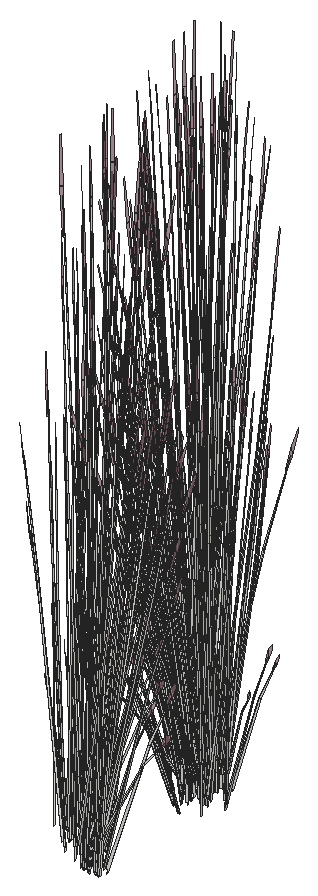
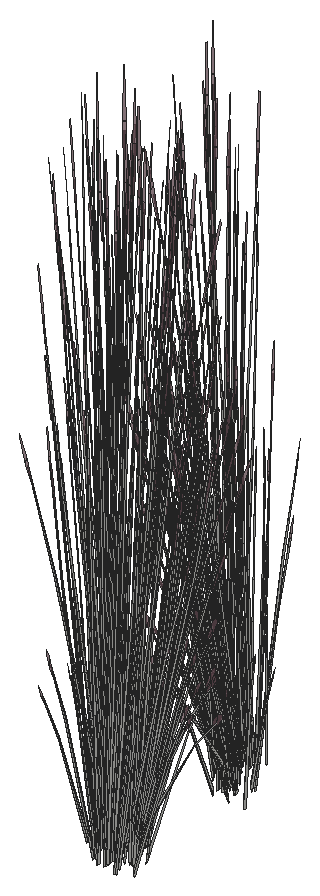
# SketchUp Ruby script. Lengths in inches.
U = 1.inch
M = Sketchup.active_model
def pt(a) = Geom::Point3d.new(a.map { |v| v * U })
def face(e, loops, mat)
  f = e.add_face(loops[0].map { |a| pt(a) })
  loops[1..].each { |l| e.add_face(l.map { |a| pt(a) }).erase! }
  f.material = f.back_material = mat if mat
  f
end
# faces: each face lists its corners as indices into pts; further lists are holes
def faces(e, pts, list, mat = nil) = list.each { |f| face(e, (f[0].is_a?(Array) ? f : [f]).map { |l| l.map { |i| pts[i] } }, mat) }
# xy, xz, yz: faces in a plane at the given z, y or x. An outline is a flat list of corners, or four numbers for a rectangle; further outlines are holes
def ring(l) = l.size == 4 ? [[l[0], l[1]], [l[2], l[1]], [l[2], l[3]], [l[0], l[3]]] : l.each_slice(2).to_a
def flat(e, list, mat, &to3) = list.each { |f| face(e, (f[0].is_a?(Array) ? f : [f]).map { |l| ring(l).map { |u, v| to3.(u, v) } }, mat) }
def xy(e, z, list, mat = nil) = flat(e, list, mat) { |x, y| [x, y, z] }
def xz(e, y, list, mat = nil) = flat(e, list, mat) { |x, z| [x, y, z] }
def yz(e, x, list, mat = nil) = flat(e, list, mat) { |y, z| [x, y, z] }
def lines(e, pts, list) = list.each { |a, b| e.add_line(pt(pts[a]), pt(pts[b])) }
# prism: a flat outline (further loops are holes) pulled along v
def prism(e, loops, v, mat = nil)
  f = face(e, loops, mat); d = Geom::Vector3d.new(v.map { |x| x * U })
  f.pushpull(f.normal.samedirection?(d) ? d.length : -d.length)
end
def box(e, o, s, mat = nil) = prism(e, [[o, [o[0] + s[0], o[1], o[2]], [o[0] + s[0], o[1] + s[1], o[2]], [o[0], o[1] + s[1], o[2]]]], [0, 0, s[2]], mat)
def at(x, y, z, deg = 0) = Geom::Transformation.translation(pt([x, y, z])) * Geom::Transformation.rotation(ORIGIN, Z_AXIS, deg.degrees)
def axes(o, x, y, z) = Geom::Transformation.new([*x, 0, *y, 0, *z, 0, *pt(o).to_a, 1])
def part(name) = M.definitions.add(name)
# library, detail: a bought-in or finely detailed component or shape, given as its bounding box
def library(name, o, s) = part(name).tap { |d| box(d.entities, o, s) }
def detail(e, o, s) = box(e.add_group.entities, o, s)
def put(e, d, t, mat = nil) = e.add_instance(d, t).tap { |i| i.material = mat if mat }
def group(e, t, mat = nil) = e.add_group.tap { |g| g.transformation = t; g.material = mat if mat }.entities
root = M.entities
M.materials.add("LightPink_Translucent").color = [144, 107, 117]
M.materials["LightPink_Translucent"].alpha = 0.75
c1 = part("blade")
p = [[2.15,0.21,22],[0,0.17,0],[0.09,0.45,0],[2.18,0.31,22],[2.29,0.31,22],[0.38,0.45,0],
  [2.48,0.24,33],[2.49,0.24,33],[2.48,0.22,33]]
faces(c1.entities,p,[[0,1,2,3],[4,5,2,3],[6,3,4,7],[8,0,3,6]])
c2 = part("seeds")
p = [[0.3,-0.1,1.38],[-0.01,-0.03,1.59],[-0.01,-0.03,0.03],[0.14,-0.07,-0.07],[0.29,-0.03,3],[0.15,0.01,3.11]]
faces(c2.entities,p,[[0,1,2,3],[1,0,4,5]],"LightPink_Translucent")
c3 = part("blade with seeds")
put(c3.entities,c1,at(0,0,0))
put(c3.entities,c2,axes([2.4,0.25,30.99],[1.5799,-0.05474,1.17369],[-0.12525,1.92788,0.29478],[-0.07173,-0.02425,1.56792]))
put(root,c3,axes([332.19,394.79,1403.03],[0.0189,-0.47427,-0.1216],[0.35781,0.01296,-0.67495],[0.13781,0.03295,1.02557]))
put(root,c3,axes([332.52,393.52,1400.48],[0,-0.46636,0.49651],[0.39487,0,0],[0,0.10622,1.57504]))
put(root,c3,axes([331.53,393.87,1400.72],[0.38326,-0.02879,0.44739],[0.03466,0.47788,-0.21531],[-0.06861,0.04843,1.43643]))
put(root,c3,axes([331.77,393.39,1400.62],[0.32884,-0.136,0.1448],[0.11516,0.38837,-0.41347],[0,0.08547,1.26744]))
put(root,c3,axes([332.14,394.6,1403.05],[-0.20082,-0.29199,0.35414],[0.2293,-0.2764,-0.4572],[0.1165,0.04206,0.87481]))
put(root,c3,axes([331.1875,394.1,1400.21],[-0.38326,0.02879,-0.44739],[-0.03466,-0.47788,0.21531],[-0.06861,0.04843,1.43643]))
put(root,c3,axes([332.99,394.33,1400.59],[-0.085,-0.1147,1.43002],[0.1106,-0.37943,-0.30754],[0.17198,0.0514,0.61141]))
put(root,c3,axes([331.47,394.75,1400.2],[0.35581,0.20937,0],[-0.17124,0.43505,0],[0,0,1.74954]))
put(root,c3,axes([332.5,394.51,1402.72],[0.07571,-0.00789,1.74944],[0.20767,-0.36231,-0.27667],[0.13467,0.04783,0.14031]))
put(root,c3,axes([331.61,395.21,1400.19],[-0.21791,-0.46895,-0.05142],[0.36918,-0.26061,0.51607],[-0.09097,0.04465,1.6363]))
put(root,c3,axes([331.53,394.08,1400.62],[0.26075,0.2802,0.1448],[-0.2175,0.31612,-0.41347],[-0.06054,0.04274,1.26744]))
put(root,c3,axes([329.47,394.15,1402.73],[-0.08753,-0.42921,0.48003],[0.34336,-0.07449,0.3958],[-0.1012,0.10094,0.9933]))
put(root,c3,axes([329.41,394.07,1402.73],[-0.2423,-0.19613,0.0643],[0.14107,-0.2793,0.50621],[-0.07768,0.0903,0.77189]))
put(root,c3,axes([329.52,393.55,1401.875],[0.12246,-0.09864,1.71376],[0.1031,0.45582,0.13857],[-0.19225,0.10302,0.73262]))
put(root,c3,axes([332.21,394.5625,1402.98],[0.35281,0.01123,-0.71045],[-0.0237,0.47284,0.08574],[0.14947,0.0499,1.00501]))
put(root,c3,axes([331.8125,394.94,1400.48],[0.33032,-0.23318,0.49651],[0.19744,0.41812,0],[-0.07523,0.05311,1.57504]))
put(root,c3,axes([331.34,394.57,1400.29],[0.15345,0.53576,-0.06012],[-0.43845,0.18773,0],[0.00536,0.01871,1.72173]))
put(root,c3,axes([331.51,395.15,1400.03],[-0.32928,-0.11539,-0.30978],[0.08291,-0.40636,0.30978],[-0.06638,0.04686,1.38974]))
put(root,c3,axes([329.14,394.33,1400.59],[0.12266,0.03828,1.43002],[0.07906,0.39104,-0.30754],[-0.16661,0.0732,0.61141]))
put(root,c3,axes([329.6875,394.01,1403.05],[0.30722,-0.06665,0.35414],[0.08112,0.381,-0.4572],[-0.08804,0.10234,0.87481]))
put(root,c3,axes([332.78,393.6,1400.375],[0.44133,0,0],[0,0.52122,-0.51607],[0,0.11871,1.63711]))
put(root,c3,axes([328.5,393.84,1402.71],[0.04504,0.01251,1.77383],[0.13934,0.41205,-0.16761],[-0.0922,0.10815,0.31391]))
put(root,c3,axes([332.61,393.87,1400.2],[-0.44111,-0.00373,-0.04976],[0,-0.52122,0.49943],[-0.01386,0.11865,1.58352]))
put(root,c3,axes([331.65,393.42,1400.67],[0.39748,0.22252,-0.29095],[-0.19139,0.46966,-0.50002],[0.01249,0.11531,1.59708]))
put(root,c3,axes([328.88,395.15,1400.77],[0.14709,-0.21136,1.1486],[0.05804,0.3346,0.84392],[-0.1063,0.05991,0.25299]))
put(root,c3,axes([332.42,394.76,1402.53],[0.20082,0.29199,-0.35414],[-0.2293,0.2764,0.4572],[0.1165,0.04206,0.87481]))
put(root,c3,axes([332.52,393.95,1400.03],[-0.24637,0.29097,-0.30978],[-0.24637,-0.29097,0.30978],[0,0.09372,1.38974]))
put(root,c3,axes([331.46,393.97,1400.67],[0.04113,0.53214,-0.29095],[-0.42835,0.03218,-0.50002],[-0.07543,0.07088,1.59708]))
put(root,c3,axes([332.32,394.87,1402.73],[-0.01777,0.35463,0.0643],[-0.26836,-0.00972,0.50621],[0.1028,0.03711,0.77189]))
put(root,c3,axes([331.61,393.77,1400.21],[-0.17124,0.42022,-0.44739],[-0.35581,-0.20224,0.21531],[0,0.09687,1.43643]))
put(root,c3,axes([329.43,394.23,1402.53],[-0.30722,0.06665,-0.35414],[-0.08112,-0.381,0.4572],[-0.08804,0.10234,0.87481]))
put(root,c3,axes([332.34,394.76,1402.73],[-0.26024,0.30729,0.48003],[-0.22444,-0.32634,0.3958],[0.1221,0.05668,0.9933]))
put(root,c3,axes([328.99,395.09,1403.65],[0.31145,0.12449,-0.06488],[-0.0958,0.38314,-0.29416],[-0.05094,0.05817,0.97024]))
put(root,c3,axes([331.2,394.38,1400.06],[-0.23773,0.35053,-0.62353],[-0.29532,-0.31785,-0.16365],[-0.09526,0.08744,1.37633]))
put(root,c3,axes([331.52,395.11,1403.05],[-0.05451,-0.37564,0.35414],[0.31161,-0.09919,-0.4572],[0.0837,0.10765,0.87481]))
put(root,c3,axes([331.62,394.97,1400.33],[0.44186,0.15158,0.30756],[-0.11054,0.54181,-0.36492],[-0.07313,0.06781,1.64885]))
put(root,c3,axes([331.59,395.34,1400.02],[-0.33032,0.23318,-0.49651],[-0.19744,-0.41812,0],[-0.07523,0.05311,1.57504]))
put(root,c3,axes([332.6875,393.96,1400.02],[0,0.46636,-0.49651],[-0.39487,0,0],[0,0.10622,1.57504]))
put(root,c3,axes([331.7,394.01,1401.875],[-0.1311,-0.08035,1.71376],[0.27131,-0.33708,0.13857],[0.16909,0.15206,0.73262]))
put(root,c3,axes([331.72,392.95,1402.47],[-0.30498,-0.24231,1.38283],[0.32203,-0.37727,0.59665],[0.0984,0.22736,1.33663]))
put(root,c3,axes([329.53,393.97,1403.03],[0.32648,0.25715,-0.1216],[-0.18809,0.3724,-0.67495],[-0.09224,0.12945,1.02557]))
put(root,c3,axes([332.18,394.92,1400.77],[-0.19872,-0.13409,1.1486],[0.2566,-0.13625,0.84392],[0.06921,0.11541,0.25299]))
put(root,c3,axes([331.49,395.31,1403.03],[0.21031,-0.39918,-0.1216],[0.30457,0.22997,-0.67495],[0.10587,0.11278,1.02557]))
put(root,c3,axes([329.97,393.86,1401.875],[0.08815,-0.14329,1.71376],[0.22258,0.38678,0.13857],[-0.15267,0.17614,0.73262]))
put(root,c3,axes([329.6875,394.28,1402.68],[0.09067,0.42583,-0.51099],[-0.34336,0.07449,-0.3958],[-0.0984,0.11438,0.97773]))
put(root,c3,axes([330.1,394.77,1403.05],[0.23881,-0.24554,0.35414],[0.22606,0.28036,-0.4572],[-0.0344,0.14245,0.87481]))
put(root,c3,axes([331.89,395.26,1400.375],[0.22066,0.46731,0],[-0.36918,0.26061,-0.51607],[-0.08408,0.05936,1.63711]))
put(root,c3,axes([331.21,395.64,1402.71],[0.00104,-0.05646,1.77383],[0.30246,-0.2491,-0.16761],[0.10506,0.08891,0.31391]))
put(root,c3,axes([332.24,395.42,1399.49],[0.02571,-0.06733,1.76342],[0.32373,-0.19829,-0.26939],[0.09815,0.10263,0.30037]))
put(root,c3,axes([331.7,393.41,1400.84],[-0.00964,-0.43909,1.41272],[0.43635,0.11382,0.59816],[-0.1032,0.24027,1.3335]))
put(root,c3,axes([331.8125,393.89,1400.09],[0.12941,0.42699,-0.69212],[-0.37279,0.15378,-0.18165],[0.0143,0.14459,1.52773]))
put(root,c3,axes([329.88,394.99,1402.73],[-0.29004,-0.02173,0.0643],[0.00795,-0.32812,0.50621],[-0.03035,0.12569,0.77189]))
put(root,c3,axes([329.27,395.36,1399.49],[0.04734,0.04659,1.76342],[0.08027,0.4317,-0.26939],[-0.10492,0.09206,0.30037]))
put(root,c3,axes([329.98,395.02,1402.73],[-0.25132,-0.3182,0.48003],[0.2669,-0.27442,0.3958],[-0.04636,0.14929,0.9933]))
put(root,c3,axes([331.74,395.11,1402.68],[0.34827,-0.11086,-0.51099],[0.06092,0.41983,-0.3958],[0.09354,0.12031,0.97773]))
put(root,c3,axes([330.77,395.17,1403.05],[0.1064,-0.35863,0.35414],[0.31043,0.1046,-0.4572],[0.02846,0.14439,0.87481]))
put(root,c3,axes([332.22,395.53,1400.67],[-0.22633,-0.01463,1.0506],[0.14947,-0.31064,0.58006],[0.08941,0.11036,0.8241]))
put(root,c3,axes([331.56,395.45,1402.73],[-0.16041,0.29625,0.0643],[-0.22843,-0.17248,0.50621],[0.07385,0.09498,0.77189]))
put(root,c3,axes([331.1875,396.45,1403.65],[0.2439,-0.26754,-0.06488],[0.22348,0.29302,-0.29416],[0.01573,0.08303,0.97024]))
put(root,c3,axes([331.63,395.37,1402.73],[-0.35104,0.10702,0.48003],[-0.06092,-0.41983,0.3958],[0.08256,0.12373,0.9933]))
put(root,c3,axes([329.9,394.21,1401.875],[0.06572,-0.16029,1.71376],[0.27569,0.33172,0.13857],[-0.12437,0.20675,0.73262]))
put(root,c3,axes([331.48,394.78,1400.59],[0.00623,-0.15459,1.43002],[0.29764,-0.17268,-0.30754],[0.09188,0.18503,0.61141]))
put(root,c3,axes([330.67,395.5,1402.73],[-0.26007,0.1585,0.0643],[-0.12729,-0.28902,0.50621],[0.02512,0.1274,0.77189]))
put(root,c3,axes([329.98,395.12,1402.53],[-0.23881,0.24554,-0.35414],[-0.22606,-0.28036,0.4572],[-0.0344,0.14245,0.87481]))
put(root,c3,axes([329.15,395.04,1402.72],[-0.00877,0.09229,1.74944],[0.24897,0.32105,-0.27667],[-0.06518,0.15182,0.14031]))
put(root,c3,axes([329.95,394.83,1403.4],[0.3879,0.02311,-0.13498],[-0.0106,0.43749,-0.74919],[-0.02694,0.1685,1.13838]))
put(root,c3,axes([330.67,395.32,1403.03],[0.34538,-0.21713,-0.1216],[0.16972,0.38536,-0.67495],[0.04557,0.16239,1.02557]))
put(root,c3,axes([330.77,395.47,1403.0625],[-0.34777,-0.12192,0.53283],[0.11892,-0.40083,0.43934],[0.0209,0.15763,1.10256]))
put(root,c3,axes([330.13,396.07,1400.77],[-0.00913,-0.2773,1.1486],[0.22824,0.19778,0.84392],[-0.04489,0.13217,0.25299]))
put(root,c3,axes([330.73,395.41,1399.49],[0.05712,-0.02538,1.76342],[0.34359,0.13968,-0.26939],[0.01005,0.15742,0.30037]))
put(root,c3,axes([330.21,395,1403],[0.25266,0.31335,-0.5672],[-0.2669,0.27442,-0.43934],[-0.03844,0.15921,1.08528]))
put(root,c3,axes([329.9375,395.47,1400.82],[0.32063,-0.08258,0.06507],[0.07371,0.33271,-0.86304],[-0.02033,0.16842,0.7736]))
put(root,c3,axes([330.96,395.3,1402.68],[0.34695,0.11691,-0.51099],[-0.11892,0.40083,-0.3958],[0.03181,0.16138,0.97773]))
put(root,c3,axes([331.16,394.48,1401.875],[-0.08068,-0.14973,1.71376],[0.3728,-0.12606,0.13857],[0.08426,0.23506,0.73262]))
put(root,c3,axes([330.8,395.55,1402.53],[-0.1064,0.35863,-0.35414],[-0.31043,-0.1046,0.4572],[0.02846,0.14439,0.87481]))
put(root,c3,axes([330.13,394.86,1403.34],[-0.00918,0.43138,-0.7886],[-0.38672,-0.02897,0.09517],[-0.04081,0.18275,1.11556]))
put(root,c3,axes([329.125,395.99,1402.71],[0.04004,-0.02816,1.77383],[0.33095,0.18728,-0.16761],[-0.00778,0.15594,0.31391]))
put(root,c3,axes([330.5,394.55,1401.875],[-0.00864,-0.17899,1.71376],[0.37441,0.11874,0.13857],[-0.02316,0.25508,0.73262]))
put(root,c3,axes([330.84,395.23,1402.98],[0.16845,0.3792,-0.71045],[-0.34676,0.21133,0.08574],[0.03939,0.18322,1.00501]))
put(root,c3,axes([329.86,395.82,1400.59],[0.11138,-0.07357,1.43002],[0.27499,0.22183,-0.30754],[-0.08185,0.19194,0.61141]))
put(root,c3,axes([330.58,396.18,1402.72],[0.04474,0.0751,1.74944],[0.36104,0.0295,-0.27667],[0.03631,0.16562,0.14031]))
put(root,c3,axes([330.01,395.46,1401.36],[0.00775,-0.24075,1.54345],[0.34877,0.12716,0.21329],[-0.03022,0.25658,0.72882]))
put(root,c3,axes([330.27,406.28,1401.875],[0.08068,0.14973,1.71376],[-0.3728,0.12606,0.13857],[-0.08426,-0.23506,0.73262]))
put(root,c3,axes([330.89,405.29,1402.72],[-0.05398,-0.06539,1.74944],[-0.36026,0.04145,-0.27667],[-0.0575,-0.15639,0.14031]))
put(root,c3,axes([331.72,406.0625,1400.59],[-0.10032,0.0944,1.43002],[-0.30046,-0.16522,-0.30754],[0.05569,-0.20547,0.61141]))
put(root,c3,axes([331.27,406.39,1402.98],[-0.16845,-0.3792,-0.71045],[0.34676,-0.21133,0.08574],[-0.03939,-0.18322,1.00501]))
put(root,c3,axes([330.17,405.88,1400.59],[-0.02137,0.15256,1.43002],[-0.31245,0.12771,-0.30754],[-0.07303,-0.19719,0.61141]))
put(root,c3,axes([330.98,405.55,1399.49],[-0.0592,0.0168,1.76342],[-0.32738,-0.18913,-0.26939],[0.00549,-0.15776,0.30037]))
put(root,c3,axes([331.97,406.76,1402.98],[0.00918,-0.43138,-0.71045],[0.38672,0.02897,0.08574],[0.04081,-0.18275,1.00501]))
put(root,c3,axes([332.51,406.09,1402.72],[-0.00341,-0.09282,1.74944],[-0.28775,-0.26825,-0.27667],[0.04449,-0.16261,0.14031]))
put(root,c3,axes([331.3,406.07,1402.53],[0.1064,-0.35863,-0.35414],[0.31043,0.1046,0.4572],[-0.02846,-0.14439,0.87481]))
put(root,c3,axes([331.53,406.54,1401.875],[-0.06572,0.16029,1.71376],[-0.27569,-0.33172,0.13857],[0.12437,-0.20675,0.73262]))
put(root,c3,axes([332.43,405.75,1402.71],[-0.03584,0.03562,1.77383],[-0.35118,-0.12018,-0.16761],[-0.01271,-0.15545,0.31391]))
put(root,c3,axes([331.14,406.31,1402.68],[-0.34695,-0.11691,-0.51099],[0.11892,-0.40083,-0.3958],[-0.03181,-0.16138,0.97773]))
put(root,c3,axes([331.35,405.3125,1400.77],[0.04528,0.27194,1.1486],[-0.25117,-0.15062,0.84392],[0.02703,-0.13924,0.25299]))
put(root,c3,axes([331.89,406.62,1402.68],[-0.25266,-0.31335,-0.51099],[0.2669,-0.27442,-0.3958],[0.03844,-0.15921,0.97773]))
put(root,c3,axes([330.52,405.07,1402.71],[-0.00658,0.0559,1.77383],[-0.32474,0.20287,-0.16761],[-0.09556,-0.1037,0.31391]))
put(root,c3,axes([330.45,406.0625,1403.09],[0.39316,-0.11987,0.53763],[0.06823,0.47021,0.4433],[-0.09247,-0.13858,1.11249]))
put(root,c3,axes([331.34,406.15,1402.73],[0.34777,0.12192,0.48003],[-0.11892,0.40083,0.3958],[-0.0209,-0.15763,0.9933]))
put(root,c3,axes([331.4375,406.3,1403.03],[-0.34538,0.21713,-0.1216],[-0.16972,-0.38536,-0.67495],[-0.04557,-0.16239,1.02557]))
put(root,c3,axes([332.15,406.78,1403.03],[-0.3879,-0.02311,-0.1216],[0.0106,-0.43749,-0.67495],[0.02694,-0.1685,1.02557]))
put(root,c3,axes([332.13,406.5,1402.53],[0.23881,-0.24554,-0.35414],[0.22606,0.28036,0.4572],[0.0344,-0.14245,0.87481]))
put(root,c3,axes([330.0625,405.64,1400.77],[0.18411,0.16231,1.1486],[-0.26813,0.09757,0.84392],[-0.05737,-0.12474,0.25299]))
put(root,c3,axes([331.43,406.12,1402.73],[0.26007,-0.1585,0.0643],[0.12729,0.28902,0.50621],[-0.02512,-0.1274,0.77189]))
put(root,c3,axes([330.51,406.5,1402.98],[-0.30095,-0.22541,-0.71045],[0.21388,-0.395,0.08574],[-0.10904,-0.13459,1.00501]))
put(root,c3,axes([330.4,406.2,1402.53],[-0.05451,-0.37564,-0.35414],[0.31161,-0.09919,0.4572],[-0.0837,-0.10765,0.87481]))
put(root,c3,axes([330.54,406.17,1402.73],[0.16041,-0.29625,0.0643],[0.22843,0.17248,0.50621],[-0.07385,-0.09498,0.77189]))
put(root,c3,axes([329.92,406.13,1399.49],[-0.03419,0.06144,1.76342],[-0.3455,0.13246,-0.26939],[-0.08346,-0.12049,0.30037]))
put(root,c3,axes([330.49,407.82,1400.1],[-0.14494,-0.47823,-0.69835],[0.41752,-0.17223,-0.18329],[-0.01602,-0.16194,1.54149]))
put(root,c3,axes([329.73,406.75,1401.875],[0.1311,0.08035,1.71376],[-0.27131,0.33708,0.13857],[-0.16909,-0.15206,0.73262]))
put(root,c3,axes([332.43,406.35,1399.49],[-0.05283,-0.03674,1.76342],[-0.13569,-0.41045,-0.26939],[0.09154,-0.11138,0.30037]))
put(root,c3,axes([331.33,406.45,1403.05],[-0.1064,0.35863,0.35414],[-0.31043,-0.1046,-0.4572],[-0.02846,-0.14439,0.87481]))
put(root,c3,axes([330.37,406.51,1402.68],[-0.34827,0.11086,-0.51099],[-0.06092,-0.41983,-0.3958],[-0.09354,-0.12031,0.97773]))
put(root,c3,axes([332.125,406.6,1402.73],[0.25132,0.3182,0.48003],[-0.2669,0.27442,0.3958],[0.04636,-0.14929,0.9933]))
put(root,c3,axes([330.61,406.14,1403.43],[-0.23555,0.44708,-0.13619],[-0.34112,-0.25757,-0.75594],[-0.11858,-0.12631,1.14864]))
put(root,c3,axes([332.22,406.63,1402.73],[0.29004,0.02173,0.0643],[-0.00795,0.32812,0.50621],[0.03035,-0.12569,0.77189]))
put(root,c3,axes([332,406.85,1403.05],[-0.23881,0.24554,0.35414],[-0.22606,-0.28036,-0.4572],[0.0344,-0.14245,0.87481]))
put(root,c3,axes([332.42,407.51,1402.98],[0.18436,-0.36797,-0.71045],[0.32306,0.26151,0.08574],[0.11008,-0.13332,1.00501]))
put(root,c3,axes([330.43,406.44,1400.375],[-0.22066,-0.46731,0],[0.36918,-0.26061,-0.51607],[0.08408,-0.05936,1.63711]))
put(root,c3,axes([332.41,407.34,1402.68],[-0.09067,-0.42583,-0.51099],[0.34336,-0.07449,-0.3958],[0.0984,-0.11438,0.97773]))
put(root,c3,axes([330.92,405.88,1400.13],[-0.2439,0.26754,-0.03893],[-0.22348,-0.29302,-0.17649],[-0.01573,-0.08303,0.58215]))
put(root,c3,axes([329.71,406.01,1402.72],[-0.07594,-0.00329,1.74944],[-0.24177,0.32918,-0.27667],[-0.129,-0.06726,0.14031]))
put(root,c3,axes([332.58,407.64,1403.03],[-0.32648,-0.25715,-0.1216],[0.18809,-0.3724,-0.67495],[0.09224,-0.12945,1.02557]))
put(root,c3,axes([331.23,409.05,1401.33],[0.305,0.18805,1.51261],[-0.29879,0.40513,0.59816],[-0.13384,-0.24012,1.26806]))
put(root,c3,axes([330.59,406.51,1403.05],[0.05451,0.37564,0.35414],[-0.31161,0.09919,-0.4572],[-0.0837,-0.10765,0.87481]))
put(root,c3,axes([329.63,407.75,1400.02],[0,-0.46636,-0.49651],[0.39487,0,0],[0,-0.10622,1.57504]))
put(root,c3,axes([330.73,406.37,1400.02],[0.33032,-0.23318,-0.49651],[0.19744,0.41812,0],[0.07523,-0.05311,1.57504]))
put(root,c3,axes([332.69,407.17,1400.59],[-0.12609,-0.01381,1.43002],[-0.12917,-0.37055,-0.30754],[0.1549,-0.10482,0.61141]))
put(root,c3,axes([329.65,406.75,1403.09],[0.29147,-0.34417,0.53763],[0.25138,0.3655,0.4433],[-0.13675,-0.06349,1.11249]))
put(root,c3,axes([333.38,407.53,1402.71],[-0.0461,-0.00354,1.77383],[-0.19143,-0.37951,-0.16761],[0.07688,-0.12478,0.31391]))
put(root,c3,axes([331.12,407.32,1400.06],[0.23773,-0.35053,-0.62353],[0.29532,0.31785,-0.16365],[0.09526,-0.08744,1.37633]))
put(root,c3,axes([332.84,406.49,1400.77],[-0.11756,0.2374,1.1486],[-0.10105,-0.31895,0.84392],[0.09709,-0.07992,0.25299]))
put(root,c3,axes([332.67,407.38,1402.53],[0.30722,-0.06665,-0.35414],[0.08112,0.381,0.4572],[0.08804,-0.10234,0.87481]))
put(root,c3,axes([329.78,406.75,1402.73],[0.01777,-0.35463,0.0643],[0.26836,0.00972,0.50621],[-0.1028,-0.03711,0.77189]))
put(root,c3,axes([330.71,407.9375,1400.21],[0.17124,-0.42022,-0.44739],[0.35581,0.20224,0.21531],[0,-0.09687,1.43643]))
put(root,c3,axes([329.68,406.86,1402.53],[-0.20082,-0.29199,-0.35414],[0.2293,-0.2764,0.4572],[-0.1165,-0.04206,0.87481]))
put(root,c3,axes([330.86,407.73,1400.67],[-0.04113,-0.53214,-0.29095],[0.42835,-0.03218,-0.50002],[0.07543,-0.07088,1.59708]))
put(root,c3,axes([329.8,407.76,1400.03],[0.24637,-0.29097,-0.30978],[0.24637,0.29097,0.30978],[0,-0.09372,1.38974]))
put(root,c3,axes([329.7,406.36,1400.13],[-0.10181,0.3808,-0.03893],[-0.31336,-0.11714,-0.17649],[-0.04758,-0.06228,0.58215]))
put(root,c3,axes([332.42,407.61,1403.05],[-0.30722,0.06665,0.35414],[-0.08112,-0.381,-0.4572],[0.08804,-0.10234,0.87481]))
put(root,c3,axes([330.67,408.29,1400.67],[-0.39748,-0.22252,-0.29095],[0.19139,-0.46966,-0.50002],[-0.01249,-0.11531,1.59708]))
put(root,c3,axes([329.53,408.1,1400.375],[-0.44133,0,0],[0,-0.52122,-0.51607],[0,-0.11871,1.63711]))
put(root,c3,axes([329.61,407.17,1400.59],[0.06891,0.12984,1.43002],[-0.15879,0.35293,-0.30754],[-0.16304,-0.08436,0.61141]))
put(root,c3,axes([330.81,406.55,1400.03],[0.32928,0.11539,-0.30978],[-0.08291,0.40636,0.30978],[0.06638,-0.04686,1.38974]))
put(root,c3,axes([329.89,407.06,1402.98],[-0.35281,-0.01123,-0.71045],[0.0237,-0.47284,0.08574],[-0.14947,-0.0499,1.00501]))
put(root,c3,axes([332.7,407.55,1402.73],[0.2423,0.19613,0.0643],[-0.14107,0.2793,0.50621],[0.07768,-0.0903,0.77189]))
put(root,c3,axes([332.63,407.47,1402.73],[0.08753,0.42921,0.48003],[-0.34336,0.07449,0.3958],[0.1012,-0.10094,0.9933]))
put(root,c3,axes([333.55,407.99,1402.72],[0.04898,-0.07104,1.74944],[-0.06269,-0.43574,-0.27667],[0.12289,-0.08262,0.14031]))
put(root,c3,axes([329.875,407.97,1400.33],[-0.32829,0.39208,0.30756],[-0.32849,-0.38796,-0.36492],[-0.01146,-0.11134,1.64885]))
put(root,c3,axes([329.42,406.29,1402.71],[0.02617,0.04654,1.77383],[-0.12614,0.41836,-0.16761],[-0.12775,0.00303,0.31391]))
put(root,c3,axes([330.92,408.15,1400.43],[0.39767,0.22603,0.24065],[-0.19139,0.46966,0.50002],[0,-0.10827,1.60543]))
put(root,c3,axes([330.77,408.78,1400.4375],[0.09355,-0.55261,-0.23429],[0.44354,0.09633,0.51271],[-0.0775,-0.07631,1.5644]))
put(root,c3,axes([329.78,407.15,1402.68],[-0.25628,0.30892,-0.51099],[-0.22444,-0.32634,-0.3958],[-0.13021,-0.047,0.97773]))
put(root,c3,axes([329.97,407.01,1403.05],[0.20082,0.29199,0.35414],[-0.2293,0.2764,-0.4572],[-0.1165,-0.04206,0.87481]))
put(root,c3,axes([329.2,407.5625,1400.77],[0.22533,-0.03337,1.1486],[-0.14293,0.29403,0.84392],[-0.11135,-0.04411,0.25299]))
put(root,c3,axes([330.79,407.83,1400.72],[-0.38326,0.02879,0.44739],[-0.03466,-0.47788,-0.21531],[0.06861,-0.04843,1.43643]))
put(root,c3,axes([329.91,406.83,1403.03],[-0.0189,0.47427,-0.1216],[-0.35781,-0.01296,-0.67495],[-0.13781,-0.03295,1.02557]))
put(root,c3,axes([329.8,408.18,1400.48],[0,0.46636,0.49651],[-0.39487,0,0],[0,-0.10622,1.57504]))
put(root,c3,axes([332.59,408.65,1403.03],[-0.17758,-0.42229,-0.1216],[0.31518,-0.20752,-0.67495],[0.13282,-0.05572,1.02557]))
put(root,c3,axes([332.57,408.29,1402.68],[0.09562,-0.42421,-0.51099],[0.32782,0.1454,-0.3958],[0.13199,-0.0389,0.97773]))
put(root,c3,axes([332.06,406.56,1400.375],[0.22066,-0.46731,0],[0.36918,0.26061,-0.51607],[0.08408,0.05936,1.63711]))
put(root,c3,axes([329.46,407.48,1401.875],[0.14639,-0.01056,1.71376],[-0.09712,0.45778,0.13857],[-0.20862,-0.02831,0.73262]))
put(root,c3,axes([330.73,408.56,1400.21],[-0.21202,-0.39143,-0.44739],[0.32115,-0.27564,0.21531],[-0.06861,-0.04843,1.43643]))
put(root,c3,axes([330.78,408.01,1400.36],[0.15345,0.52148,0.45755],[-0.43845,0.18134,0.17955],[0.00536,-0.09582,1.58856]))
put(root,c3,axes([332.92,408.41,1399.98],[-0.22732,0.05597,1.41583],[-0.03618,-0.44548,0.08104],[0.15921,-0.06743,0.80566]))
put(root,c3,axes([333.34,408.01,1400.26],[-0.21881,-0.29821,-0.06488],[0.23965,-0.27324,-0.29416],[0.0679,-0.01924,0.97024]))
put(root,c3,axes([330.7,408.42,1400.72],[-0.17124,0.42022,0.44739],[-0.35581,-0.20224,-0.21531],[0,-0.09687,1.43643]))
put(root,c3,axes([331.33,408.05,1400.21],[0,-0.53961,0],[0.44133,0,0],[0,0,1.79456]))
put(root,c3,axes([331.87,406.8,1400.48],[-0.33032,-0.23318,0.49651],[0.19744,-0.41812,0],[0.07523,0.05311,1.57504]))
put(root,c3,axes([332.51,408.44,1402.98],[0.31014,-0.20596,-0.71045],[0.17284,0.42397,0.08574],[0.14985,-0.04816,1.00501]))
put(root,c3,axes([330.54,408.71,1400.06],[-0.36714,-0.07646,-0.62353],[0.07747,-0.47163,-0.16365],[-0.10956,-0.05715,1.37633]))
put(root,c3,axes([331.12,407.71,1400.36],[-0.29264,0.42323,0.45755],[-0.34767,-0.3736,0.17955],[0.07055,-0.04224,1.58856]))
put(root,c3,axes([331.44,408.47,1400.3],[-0.32829,-0.4014,-0.06131],[0.32849,-0.40164,0],[-0.01146,-0.01402,1.75571]))
put(root,c3,axes([330.61,407.01,1400.47],[-0.10196,0.46348,0.17642],[-0.3731,-0.13116,0.35086],[0.06445,-0.00226,1.60407]))
put(root,c3,axes([332.47,408.52,1403.05],[-0.29332,-0.1301,0.35414],[0.08555,-0.37955,-0.4572],[0.11809,-0.0348,0.87481]))
put(root,c3,axes([329.4,407.83,1402.73],[0.09971,-0.42522,0.48003],[0.32782,0.1454,0.3958],[-0.12892,0.02555,0.9933]))
put(root,c3,axes([330.46,407.39,1399.59],[-0.3474,0.18671,1.28929],[-0.11057,-0.53572,0.50096],[0.21332,0.00891,1.46642]))
put(root,c3,axes([331.39,407.53,1400.62],[0.06809,-0.4162,0.1448],[0.33266,0.07225,-0.41347],[0.06054,0.04274,1.26744]))
put(root,c3,axes([329.37,407.71,1402.73],[-0.12963,-0.31798,0.0643],[0.23638,-0.15564,0.50621],[-0.1042,0.03071,0.77189]))
put(root,c3,axes([330.82,408.52,1400.36],[0.44609,0.09826,0.45755],[-0.09078,0.55493,0.17955],[-0.06519,-0.05359,1.58856]))
put(root,c3,axes([333.17,408.11,1399.49],[-0.01845,-0.0708,1.76342],[0.12793,-0.41416,-0.26939],[0.12905,-0.00596,0.30037]))
put(root,c3,axes([329.36,408.04,1399.49],[0.00895,0.0735,1.76342],[-0.18044,0.38382,-0.26939],[-0.12817,-0.01935,0.30037]))
put(root,c3,axes([331.25,407.64,1400.72],[-0.21202,-0.39143,0.44739],[0.32115,-0.27564,-0.21531],[0.06861,0.04843,1.43643]))
put(root,c3,axes([330.15,409.43,1400.03],[-0.08291,-0.40636,-0.30978],[0.32928,-0.11539,0.30978],[-0.06638,-0.04686,1.38974]))
put(root,c3,axes([330.58,409.4,1400.47],[0.37926,-0.12378,0.17642],[0.09365,0.46065,0.35086],[-0.03382,-0.06712,1.60407]))
put(root,c3,axes([331.36,407.66,1400.67],[0.35635,-0.30962,-0.29095],[0.23697,0.43749,-0.50002],[0.08792,0.04443,1.59708]))
put(root,c3,axes([332.78,408.48,1402.53],[0.29332,0.1301,-0.35414],[-0.08555,0.37955,0.4572],[0.11809,-0.0348,0.87481]))
put(root,c3,axes([330.0625,409.6,1400.02],[-0.33032,-0.23318,-0.49651],[0.19744,-0.41812,0],[-0.07523,-0.05311,1.57504]))
put(root,c3,axes([332.26,406.84,1400.02],[0.33032,0.23318,-0.49651],[-0.19744,0.41812,0],[0.07523,0.05311,1.57504]))
put(root,c3,axes([329.33,407.875,1402.53],[-0.29332,-0.1301,-0.35414],[0.08555,-0.37955,0.4572],[-0.11809,0.0348,0.87481]))
put(root,c3,axes([331.63,408.17,1400.21],[0.39487,0,0],[0,0.48281,0],[0,0,1.78407]))
put(root,c3,axes([330.96,408.78,1400.67],[-0.35635,0.30962,-0.29095],[-0.23697,-0.43749,-0.50002],[-0.08792,-0.04443,1.59708]))
put(root,c3,axes([331.74,407.04,1400.47],[-0.37926,0.12378,0.17642],[-0.09365,-0.46065,0.35086],[0.03382,0.06712,1.60407]))
put(root,c3,axes([331.98,408.01,1401.875],[-0.14639,0.01056,1.71376],[0.09712,-0.45778,0.13857],[0.20862,0.02831,0.73262]))
put(root,c3,axes([332.17,407.01,1400.03],[0.08291,0.40636,-0.30978],[-0.32928,0.11539,0.30978],[0.06638,0.04686,1.38974]))
put(root,c3,axes([332.73,408.64,1402.73],[0.12963,0.31798,0.0643],[-0.23638,0.15564,0.50621],[0.1042,-0.03071,0.77189]))
put(root,c3,axes([331.5,407.92,1400.38],[-0.44609,-0.09826,0.49198],[0.09078,-0.55493,0.19306],[0.06519,0.05359,1.70813]))
put(root,c3,axes([332.71,408.53,1402.73],[-0.09971,0.42522,0.48003],[-0.32782,-0.1454,0.3958],[0.12892,-0.02555,0.9933]))
put(root,c3,axes([331.15,409.29,1400.2],[-0.11516,-0.40207,0],[0.32884,-0.1408,0],[0,0,1.54371]))
put(root,c3,axes([330.93,408.91,1400.62],[-0.06809,0.4162,0.1448],[-0.33266,-0.07225,-0.41347],[-0.06054,-0.04274,1.26744]))
put(root,c3,axes([329.64,407.83,1403.05],[0.29332,0.1301,0.35414],[-0.08555,0.37955,-0.4572],[-0.11809,0.0348,0.87481]))
put(root,c3,axes([331.58,409.24,1400.18],[0.37054,-0.15823,-0.19198],[0.1302,0.45581,0.00008],[0.0409,-0.01749,1.73897]))
put(root,c3,axes([331.71,409.43,1400.47],[0.10196,-0.46348,0.17642],[0.3731,0.13116,0.35086],[-0.06445,0.00226,1.60407]))
put(root,c3,axes([331.62,408.375,1400.21],[0.24637,0.30123,0],[-0.24637,0.30123,0],[0,0,1.69266]))
put(root,c3,axes([330.22,407.8125,1401.34],[0.10032,-0.06746,1.77064],[0.0346,0.47103,0.13857],[-0.2173,0.0625,0.63284]))
put(root,c3,axes([332.29,408.25,1400.47],[-0.2773,-0.3397,0.17642],[0.27945,-0.32949,0.35086],[-0.03063,0.06937,1.60407]))
put(root,c3,axes([331.78,407.73,1400.06],[0.36714,0.07646,-0.62353],[-0.07747,0.47163,-0.16365],[0.10956,0.05715,1.37633]))
put(root,c3,axes([333.4,408.56,1400.77],[-0.21807,0.07699,1.1486],[0.10265,-0.31819,0.84392],[0.11568,0.02177,0.25299]))
put(root,c3,axes([331.07,409.48,1400.2],[-0.35581,-0.20937,0],[0.17124,-0.43505,0],[0,0,1.62707]))
put(root,c3,axes([331.36,408.92,1400.46],[-0.34464,-0.37536,-0.25192],[0.29,-0.42149,0.5513],[-0.0928,0.04391,1.68216]))
